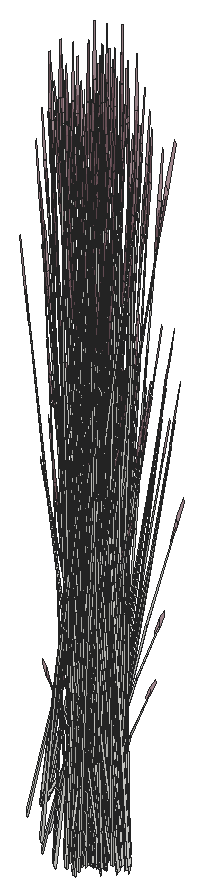
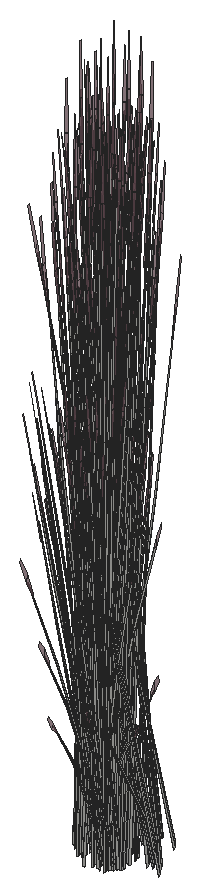
# SketchUp Ruby script. Lengths in inches.
U = 1.inch
M = Sketchup.active_model
def pt(a) = Geom::Point3d.new(a.map { |v| v * U })
def face(e, loops, mat)
  f = e.add_face(loops[0].map { |a| pt(a) })
  loops[1..].each { |l| e.add_face(l.map { |a| pt(a) }).erase! }
  f.material = f.back_material = mat if mat
  f
end
# faces: each face lists its corners as indices into pts; further lists are holes
def faces(e, pts, list, mat = nil) = list.each { |f| face(e, (f[0].is_a?(Array) ? f : [f]).map { |l| l.map { |i| pts[i] } }, mat) }
# xy, xz, yz: faces in a plane at the given z, y or x. An outline is a flat list of corners, or four numbers for a rectangle; further outlines are holes
def ring(l) = l.size == 4 ? [[l[0], l[1]], [l[2], l[1]], [l[2], l[3]], [l[0], l[3]]] : l.each_slice(2).to_a
def flat(e, list, mat, &to3) = list.each { |f| face(e, (f[0].is_a?(Array) ? f : [f]).map { |l| ring(l).map { |u, v| to3.(u, v) } }, mat) }
def xy(e, z, list, mat = nil) = flat(e, list, mat) { |x, y| [x, y, z] }
def xz(e, y, list, mat = nil) = flat(e, list, mat) { |x, z| [x, y, z] }
def yz(e, x, list, mat = nil) = flat(e, list, mat) { |y, z| [x, y, z] }
def lines(e, pts, list) = list.each { |a, b| e.add_line(pt(pts[a]), pt(pts[b])) }
# prism: a flat outline (further loops are holes) pulled along v
def prism(e, loops, v, mat = nil)
  f = face(e, loops, mat); d = Geom::Vector3d.new(v.map { |x| x * U })
  f.pushpull(f.normal.samedirection?(d) ? d.length : -d.length)
end
def box(e, o, s, mat = nil) = prism(e, [[o, [o[0] + s[0], o[1], o[2]], [o[0] + s[0], o[1] + s[1], o[2]], [o[0], o[1] + s[1], o[2]]]], [0, 0, s[2]], mat)
def at(x, y, z, deg = 0) = Geom::Transformation.translation(pt([x, y, z])) * Geom::Transformation.rotation(ORIGIN, Z_AXIS, deg.degrees)
def axes(o, x, y, z) = Geom::Transformation.new([*x, 0, *y, 0, *z, 0, *pt(o).to_a, 1])
def part(name) = M.definitions.add(name)
# library, detail: a bought-in or finely detailed component or shape, given as its bounding box
def library(name, o, s) = part(name).tap { |d| box(d.entities, o, s) }
def detail(e, o, s) = box(e.add_group.entities, o, s)
def put(e, d, t, mat = nil) = e.add_instance(d, t).tap { |i| i.material = mat if mat }
def group(e, t, mat = nil) = e.add_group.tap { |g| g.transformation = t; g.material = mat if mat }.entities
root = M.entities
M.materials.add("LightPink_Translucent").color = [144, 107, 117]
M.materials["LightPink_Translucent"].alpha = 0.75
c1 = part("blade")
p = [[2.15,0.21,22],[0,0.17,0],[0.09,0.45,0],[2.18,0.31,22],[2.29,0.31,22],[0.38,0.45,0],
  [2.48,0.24,33],[2.49,0.24,33],[2.48,0.22,33]]
faces(c1.entities,p,[[0,1,2,3],[4,5,2,3],[6,3,4,7],[8,0,3,6]])
c2 = part("seeds")
p = [[0.3,-0.1,1.38],[-0.01,-0.03,1.59],[-0.01,-0.03,0.03],[0.14,-0.07,-0.07],[0.29,-0.03,3],[0.15,0.01,3.11]]
faces(c2.entities,p,[[0,1,2,3],[1,0,4,5]],"LightPink_Translucent")
c3 = part("blade with seeds")
put(c3.entities,c1,at(0,0,0))
put(c3.entities,c2,axes([2.4,0.25,30.99],[1.5799,-0.05474,1.17369],[-0.12525,1.92788,0.29478],[-0.07173,-0.02425,1.56792]))
put(root,c3,axes([340.1,651.66,621.58],[0.44609,0.09826,0.45755],[-0.09078,0.55493,0.17955],[-0.06519,-0.05359,1.58856]))
put(root,c3,axes([337.55,651.78,624.45],[0.12963,0.31798,0.0643],[-0.23638,0.15564,0.50621],[0.1042,-0.03071,0.77189]))
put(root,c3,axes([337.24,652.63,624.25],[0.20082,0.29199,-0.35414],[-0.2293,0.2764,0.4572],[0.1165,0.04206,0.87481]))
put(root,c3,axes([341.33,650.97,624.76],[0.29332,0.1301,0.35414],[-0.08555,0.37955,-0.4572],[-0.11809,0.0348,0.87481]))
put(root,c3,axes([341.72,652.06,621.78],[-0.34464,-0.37536,-0.25192],[0.29,-0.42149,0.5513],[-0.0928,0.04391,1.68216]))
put(root,c3,axes([337.01,652.66,624.76],[0.0189,-0.47427,-0.1216],[0.35781,0.01296,-0.67495],[0.13781,0.03295,1.02557]))
put(root,c3,axes([337.53,651.66,624.46],[-0.09971,0.42522,0.48003],[-0.32782,-0.1454,0.3958],[0.12892,-0.02555,0.9933]))
put(root,c3,axes([341.38,652.15,624.39],[0.09067,0.42583,-0.51099],[-0.34336,0.07449,-0.3958],[-0.0984,0.11438,0.97773]))
put(root,c3,axes([339.98,651.55,621.94],[-0.17124,0.42022,0.44739],[-0.35581,-0.20224,-0.21531],[0,-0.09687,1.43643]))
put(root,c3,axes([342.24,651.85,621.77],[-0.36714,-0.07646,-0.62353],[0.07747,-0.47163,-0.16365],[-0.10956,-0.05715,1.37633]))
put(root,c3,axes([341.54,651.98,621.53],[-0.38326,0.02879,-0.44739],[-0.03466,-0.47788,0.21531],[-0.06861,0.04843,1.43643]))
put(root,c3,axes([339.86,652.54,621.7],[0.37926,-0.12378,0.17642],[0.09365,0.46065,0.35086],[-0.03382,-0.06712,1.60407]))
put(root,c3,axes([343.14,651.43,623.6],[0.12246,-0.09864,1.71376],[0.1031,0.45582,0.13857],[-0.19225,0.10302,0.73262]))
put(root,c3,axes([340.35,652.61,621.42],[-0.35581,-0.20937,0],[0.17124,-0.43505,0],[0,0,1.62707]))
put(root,c3,axes([340.8125,652.78,621.8],[0.33032,0.23318,0.49651],[-0.19744,0.41812,0],[-0.07523,-0.05311,1.57504]))
put(root,c3,axes([341.17,653.14,621.6],[0.22066,0.46731,0],[-0.36918,0.26061,-0.51607],[-0.08408,0.05936,1.63711]))
put(root,c3,axes([337.32,652.38,624.4375],[0.07571,-0.00789,1.74944],[0.20767,-0.36231,-0.27667],[0.13467,0.04783,0.14031]))
put(root,c3,axes([342.76,652.2,622.32],[0.12266,0.03828,1.43002],[0.07906,0.39104,-0.30754],[-0.16661,0.0732,0.61141]))
put(root,c3,axes([341.76,652.74,621.72],[-0.33032,-0.23318,-0.49651],[0.19744,-0.41812,0],[-0.07523,-0.05311,1.57504]))
put(root,c3,axes([341.22,651.85,624.74],[0.32648,0.25715,-0.1216],[-0.18809,0.3724,-0.67495],[-0.09224,0.12945,1.02557]))
put(root,c3,axes([338.22,651.7,622.49],[-0.21807,0.07699,1.1486],[0.10265,-0.31819,0.84392],[0.11568,0.02177,0.25299]))
put(root,c3,axes([341.28,652.05,621.93],[-0.06809,0.4162,0.1448],[-0.33266,-0.07225,-0.41347],[-0.06054,-0.04274,1.26744]))
put(root,c3,axes([341.96,653.02,622.08],[-0.22066,0.46731,0],[-0.36918,-0.26061,-0.51607],[-0.08408,-0.05936,1.63711]))
put(root,c3,axes([340.99,652.57,621.7],[0.10196,-0.46348,0.17642],[0.3731,0.13116,0.35086],[-0.06445,0.00226,1.60407]))
put(root,c3,axes([340.8125,651.95,621.84],[0.26075,0.2802,0.1448],[-0.2175,0.31612,-0.41347],[-0.06054,0.04274,1.26744]))
put(root,c3,axes([343.85,650.95,623.07],[0.10032,-0.06746,1.77064],[0.0346,0.47103,0.13857],[-0.2173,0.0625,0.63284]))
put(root,c3,axes([341.95,653.21,621.33],[-0.33032,0.23318,-0.49651],[-0.19744,-0.41812,0],[-0.07523,0.05311,1.57504]))
put(root,c3,axes([341.97,653.09,621.51],[-0.21791,-0.46895,-0.05142],[0.36918,-0.26061,0.51607],[-0.09097,0.04465,1.6363]))
put(root,c3,axes([340.72,651.61,621.52],[-0.32829,-0.4014,-0.06131],[0.32849,-0.40164,0],[-0.01146,-0.01402,1.75571]))
put(root,c3,axes([340.81,651.75,621.94],[0.38326,-0.02879,0.44739],[0.03466,0.47788,-0.21531],[-0.06861,0.04843,1.43643]))
put(root,c3,axes([337.59,651.62,624.25],[0.29332,0.1301,-0.35414],[-0.08555,0.37955,0.4572],[0.11809,-0.0348,0.87481]))
put(root,c3,axes([340.68,652.96,625.35],[0.31145,0.12449,-0.06488],[-0.0958,0.38314,-0.29416],[-0.05094,0.05817,0.97024]))
put(root,c3,axes([340.9,652.85,621.55],[0.44186,0.15158,0.30756],[-0.11054,0.54181,-0.36492],[-0.07313,0.06781,1.64885]))
put(root,c3,axes([341.87,653.03,621.35],[-0.32928,-0.11539,-0.30978],[0.08291,-0.40636,0.30978],[-0.06638,0.04686,1.38974]))
put(root,c3,axes([340.46,652.64,624.37],[0.23881,-0.24554,0.35414],[0.22606,0.28036,-0.4572],[-0.0344,0.14245,0.87481]))
put(root,c3,axes([337.03,652.4375,624.71],[0.35281,0.01123,-0.71045],[-0.0237,0.47284,0.08574],[0.14947,0.0499,1.00501]))
put(root,c3,axes([341.38,651.88,624.76],[0.30722,-0.06665,0.35414],[0.08112,0.381,-0.4572],[-0.08804,0.10234,0.87481]))
put(root,c3,axes([341.09,652.82,621.7],[0.33032,-0.23318,0.49651],[0.19744,0.41812,0],[-0.07523,0.05311,1.57504]))
put(root,c3,axes([342.06,651.29,622.16],[-0.00964,-0.43909,1.41272],[0.43635,0.11382,0.59816],[-0.1032,0.24027,1.3335]))
put(root,c3,axes([337.74,651.54,621.71],[-0.22732,0.05597,1.41583],[-0.03618,-0.44548,0.08104],[0.15921,-0.06743,0.80566]))
put(root,c3,axes([342.77,651.27,624.44],[-0.05763,0.06055,1.74944],[0.0049,0.44239,-0.27667],[-0.13211,0.05753,0.14031]))
put(root,c3,axes([340.43,652.43,621.43],[-0.11516,-0.40207,0],[0.32884,-0.1408,0],[0,0,1.54371]))
put(root,c3,axes([337.99,651.25,621.22],[-0.01845,-0.0708,1.76342],[0.12793,-0.41416,-0.26939],[0.12905,-0.00596,0.30037]))
put(root,c3,axes([338.12,653.04,624.43],[-0.03191,-0.04083,1.77383],[0.06981,-0.43764,-0.16761],[0.12571,-0.02796,0.31391]))
put(root,c3,axes([336.8,651.15,623.6],[-0.14639,0.01056,1.71376],[0.09712,-0.45778,0.13857],[0.20862,0.02831,0.73262]))
put(root,c3,axes([342.95,651.01,624.25],[-0.29332,-0.1301,-0.35414],[0.08555,-0.37955,0.4572],[-0.11809,0.0348,0.87481]))
put(root,c3,axes([341.8125,651.85,621.98],[0.04113,0.53214,-0.29095],[-0.42835,0.03218,-0.50002],[-0.07543,0.07088,1.59708]))
put(root,c3,axes([342.65,651.92,622.375],[-0.35635,0.30962,-0.29095],[-0.23697,-0.43749,-0.50002],[-0.08792,-0.04443,1.59708]))
put(root,c3,axes([341.67,652.89,624.44],[-0.25132,-0.3182,0.48003],[0.2669,-0.27442,0.3958],[-0.04636,0.14929,0.9933]))
put(root,c3,axes([337.33,651.58,624.71],[0.31014,-0.20596,-0.71045],[0.17284,0.42397,0.08574],[0.14985,-0.04816,1.00501]))
put(root,c3,axes([342.13,651.71,624.43],[0.04504,0.01251,1.77383],[0.13934,0.41205,-0.16761],[-0.0922,0.10815,0.31391]))
put(root,c3,axes([343.15,651.21,624.41],[-0.09562,0.42421,-0.51099],[-0.32782,-0.1454,-0.3958],[-0.13199,0.0389,0.97773]))
put(root,c3,axes([340.89,651.64,621.43],[-0.17124,0.42022,-0.44739],[-0.35581,-0.20224,0.21531],[0,0.09687,1.43643]))
put(root,c3,axes([341.85,652.57,621.74],[-0.08291,-0.40636,-0.30978],[0.32928,-0.11539,0.30978],[-0.06638,-0.04686,1.38974]))
put(root,c3,axes([341.58,652.86,624.4375],[-0.29004,-0.02173,0.0643],[0.00795,-0.32812,0.50621],[-0.03035,0.12569,0.77189]))
put(root,c3,axes([341.17,651.66,621.68],[0.44609,0.09826,0.45755],[-0.09078,0.55493,0.17955],[-0.06519,-0.05359,1.58856]))
put(root,c3,axes([342.99,651.18,621.22],[0.00895,0.0735,1.76342],[-0.18044,0.38382,-0.26939],[-0.12817,-0.01935,0.30037]))
put(root,c3,axes([341.57,651.38,621.7],[-0.2773,-0.3397,0.17642],[0.27945,-0.32949,0.35086],[-0.03063,0.06937,1.60407]))
put(root,c3,axes([340.61,651.1875,621.43],[0,-0.53961,0],[0.44133,0,0],[0,0,1.79456]))
put(root,c3,axes([341.06,651.55,622.04],[-0.17124,0.42022,0.44739],[-0.35581,-0.20224,-0.21531],[0,-0.09687,1.43643]))
put(root,c3,axes([340.83,651.4,621.52],[0,0.53934,-0.05637],[-0.44133,0,0],[0,0.01695,1.79368]))
put(root,c3,axes([342.89,652.25,621.77],[-0.23773,0.35053,-0.62353],[-0.29532,-0.31785,-0.16365],[-0.09526,0.08744,1.37633]))
put(root,c3,axes([340.05,653.05,624.28],[0.1064,-0.35863,0.35414],[0.31043,0.1046,-0.4572],[0.02846,0.14439,0.87481]))
put(root,c3,axes([342.51,653.02,622.49],[0.14709,-0.21136,1.1486],[0.05804,0.3346,0.84392],[-0.1063,0.05991,0.25299]))
put(root,c3,axes([337.81,652.21,622.31],[-0.085,-0.1147,1.43002],[0.1106,-0.37943,-0.30754],[0.17198,0.0514,0.61141]))
put(root,c3,axes([339.89,650.15,621.7],[-0.10196,0.46348,0.17642],[-0.3731,-0.13116,0.35086],[0.06445,-0.00226,1.60407]))
put(root,c3,axes([340.62,652.45,621.52],[0.15345,0.53576,-0.06012],[-0.43845,0.18773,0],[0.00536,0.01871,1.72173]))
put(root,c3,axes([340.94,652.54,621.79],[0.37926,-0.12378,0.17642],[0.09365,0.46065,0.35086],[-0.03382,-0.06712,1.60407]))
put(root,c3,axes([343.02,650.97,624.46],[0.09971,-0.42522,0.48003],[0.32782,0.1454,0.3958],[-0.12892,0.02555,0.9933]))
put(root,c3,axes([343.14,650.84,624.76],[0.17758,0.42229,-0.1216],[-0.31518,0.20752,-0.67495],[-0.13282,0.05572,1.02557]))
put(root,c3,axes([343.05,652.06,622.17],[-0.34464,-0.37536,-0.25192],[0.29,-0.42149,0.5513],[-0.0928,0.04391,1.68216]))
put(root,c3,axes([341.42,652.61,621.51],[-0.35581,-0.20937,0],[0.17124,-0.43505,0],[0,0,1.62707]))
put(root,c3,axes([342.25,653.14,621.69],[0.22066,0.46731,0],[-0.36918,0.26061,-0.51607],[-0.08408,0.05936,1.63711]))
put(root,c3,axes([343,650.85,624.46],[-0.12963,-0.31798,0.0643],[0.23638,-0.15564,0.50621],[-0.1042,0.03071,0.77189]))
put(root,c3,axes([343.59,651.73,623.6],[0.08815,-0.14329,1.71376],[0.22258,0.38678,0.13857],[-0.15267,0.17614,0.73262]))
put(root,c3,axes([341.89,651.74,621.42],[-0.44111,-0.00373,-0.04976],[0,-0.52122,0.49943],[-0.01386,0.11865,1.58352]))
put(root,c3,axes([343.0625,652.11,624.25],[-0.30722,0.06665,-0.35414],[-0.08112,-0.381,0.4572],[-0.08804,0.10234,0.87481]))
put(root,c3,axes([341.02,650.18,621.7],[-0.37926,0.12378,0.17642],[-0.09365,-0.46065,0.35086],[0.03382,0.06712,1.60407]))
put(root,c3,axes([342.88,651.98,621.92],[-0.38326,0.02879,-0.44739],[-0.03466,-0.47788,0.21531],[-0.06861,0.04843,1.43643]))
put(root,c3,axes([342.89,653.24,621.22],[0.04734,0.04659,1.76342],[0.08027,0.4317,-0.26939],[-0.10492,0.09206,0.30037]))
put(root,c3,axes([342.0625,652.57,621.79],[0.10196,-0.46348,0.17642],[0.3731,0.13116,0.35086],[-0.06445,0.00226,1.60407]))
put(root,c3,axes([341.89,651.95,621.93],[0.26075,0.2802,0.1448],[-0.2175,0.31612,-0.41347],[-0.06054,0.04274,1.26744]))
put(root,c3,axes([340.47,654.32,624.87],[0.2439,-0.26754,-0.06488],[0.22348,0.29302,-0.29416],[0.01573,0.08303,0.97024]))
put(root,c3,axes([340.4,650.85,621.58],[-0.29264,0.42323,0.45755],[-0.34767,-0.3736,0.17955],[0.07055,-0.04224,1.58856]))
put(root,c3,axes([341.8,651.61,621.61],[-0.32829,-0.4014,-0.06131],[0.32849,-0.40164,0],[-0.01146,-0.01402,1.75571]))
put(root,c3,axes([341.89,651.75,622.04],[0.38326,-0.02879,0.44739],[0.03466,0.47788,-0.21531],[-0.06861,0.04843,1.43643]))
put(root,c3,axes([340.9,651.52,621.4375],[0.24637,0.30123,0],[-0.24637,0.30123,0],[0,0,1.69266]))
put(root,c3,axes([343.1,652.03,624.46],[-0.08753,-0.42921,0.48003],[0.34336,-0.07449,0.3958],[-0.1012,0.10094,0.9933]))
put(root,c3,axes([340.9,651.16,621.94],[0.17124,-0.42022,0.44739],[0.35581,0.20224,-0.21531],[0,0.09687,1.43643]))
put(root,c3,axes([342.15,652.78,622.1875],[0.33032,0.23318,0.49651],[-0.19744,0.41812,0],[-0.07523,-0.05311,1.57504]))
put(root,c3,axes([340.75,652.62,621.43],[0.35581,0.20937,0],[-0.17124,0.43505,0],[0,0,1.74954]))
put(root,c3,axes([341.98,652.85,621.65],[0.44186,0.15158,0.30756],[-0.11054,0.54181,-0.36492],[-0.07313,0.06781,1.64885]))
put(root,c3,axes([343.03,651.94,624.46],[-0.2423,-0.19613,0.0643],[0.14107,-0.2793,0.50621],[-0.07768,0.0903,0.77189]))
put(root,c3,axes([342.17,652.82,621.8],[0.33032,-0.23318,0.49651],[0.19744,0.41812,0],[-0.07523,0.05311,1.57504]))
put(root,c3,axes([340.78,651.0625,621.61],[-0.44609,-0.09826,0.49198],[0.09078,-0.55493,0.19306],[0.06519,0.05359,1.70813]))
put(root,c3,axes([342.62,652.05,622.32],[-0.06809,0.4162,0.1448],[-0.33266,-0.07225,-0.41347],[-0.06054,-0.04274,1.26744]))
put(root,c3,axes([341.8,651.82,621.25],[-0.24637,0.29097,-0.30978],[-0.24637,-0.29097,0.30978],[0,0.09372,1.38974]))
put(root,c3,axes([343.28,653.21,621.72],[-0.33032,0.23318,-0.49651],[-0.19744,-0.41812,0],[-0.07523,0.05311,1.57504]))
put(root,c3,axes([341.5,652.43,621.52],[-0.11516,-0.40207,0],[0.32884,-0.1408,0],[0,0,1.54371]))
put(root,c3,axes([343.3,653.09,621.9],[-0.21791,-0.46895,-0.05142],[0.36918,-0.26061,0.51607],[-0.09097,0.04465,1.6363]))
put(root,c3,axes([343.53,652.09,623.6],[0.06572,-0.16029,1.71376],[0.27569,0.33172,0.13857],[-0.12437,0.20675,0.73262]))
put(root,c3,axes([341.09,651.77,621.32],[0.12941,0.42699,-0.69212],[-0.37279,0.15378,-0.18165],[0.0143,0.14459,1.52773]))
put(root,c3,axes([340.91,651.31,621.43],[0.39487,0,0],[0,0.48281,0],[0,0,1.78407]))
put(root,c3,axes([343.26,650.97,624.78],[0.29332,0.1301,0.35414],[-0.08555,0.37955,-0.4572],[-0.11809,0.0348,0.87481]))
put(root,c3,axes([340.53,650.78,621.94],[-0.21202,-0.39143,0.44739],[0.32115,-0.27564,-0.21531],[0.06861,0.04843,1.43643]))
put(root,c3,axes([343.2,653.03,621.74],[-0.32928,-0.11539,-0.30978],[0.08291,-0.40636,0.30978],[-0.06638,0.04686,1.38974]))
put(root,c3,axes([341.05,651.26,621.84],[0.32884,-0.136,0.1448],[0.11516,0.38837,-0.41347],[0,0.08547,1.26744]))
put(root,c3,axes([341.79,652.64,624.76],[0.23881,-0.24554,0.35414],[0.22606,0.28036,-0.4572],[-0.0344,0.14245,0.87481]))
put(root,c3,axes([343.3125,652.15,624.41],[0.09067,0.42583,-0.51099],[-0.34336,0.07449,-0.3958],[-0.0984,0.11438,0.97773]))
put(root,c3,axes([343.39,651.29,622.55],[-0.00964,-0.43909,1.41272],[0.43635,0.11382,0.59816],[-0.1032,0.24027,1.3335]))
put(root,c3,axes([341.97,651.64,621.53],[-0.17124,0.42022,-0.44739],[-0.35581,-0.20224,0.21531],[0,0.09687,1.43643]))
put(root,c3,axes([344.17,651.85,621.78],[-0.36714,-0.07646,-0.62353],[0.07747,-0.47163,-0.16365],[-0.10956,-0.05715,1.37633]))
put(root,c3,axes([340.93,651.29,621.89],[0.39748,0.22252,-0.29095],[-0.19139,0.46966,-0.50002],[0.01249,0.11531,1.59708]))
put(root,c3,axes([342.65,651.38,621.79],[-0.2773,-0.3397,0.17642],[0.27945,-0.32949,0.35086],[-0.03063,0.06937,1.60407]))
put(root,c3,axes([343.15,651.85,622.375],[0.04113,0.53214,-0.29095],[-0.42835,0.03218,-0.50002],[-0.07543,0.07088,1.59708]))
put(root,c3,axes([341.6875,651.1875,621.52],[0,-0.53961,0],[0.44133,0,0],[0,0,1.79456]))
put(root,c3,axes([341.91,651.4,621.61],[0,0.53934,-0.05637],[-0.44133,0,0],[0,0.01695,1.79368]))
put(root,c3,axes([341.13,653.05,624.37],[0.1064,-0.35863,0.35414],[0.31043,0.1046,-0.4572],[0.02846,0.14439,0.87481]))
put(root,c3,axes([341.8,651.4,621.7],[0,-0.46636,0.49651],[0.39487,0,0],[0,0.10622,1.57504]))
put(root,c3,axes([341.97,651.83,621.24],[0,0.46636,-0.49651],[-0.39487,0,0],[0,0.10622,1.57504]))
put(root,c3,axes([340.91,653.24,623.96],[-0.35104,0.10702,0.48003],[-0.06092,-0.41983,0.3958],[0.08256,0.12373,0.9933]))
put(root,c3,axes([343.6875,652.74,621.74],[-0.33032,-0.23318,-0.49651],[0.19744,-0.41812,0],[-0.07523,-0.05311,1.57504]))
put(root,c3,axes([340.84,653.33,623.95],[-0.16041,0.29625,0.0643],[-0.22843,-0.17248,0.50621],[0.07385,0.09498,0.77189]))
put(root,c3,axes([340.97,650.15,621.79],[-0.10196,0.46348,0.17642],[-0.3731,-0.13116,0.35086],[0.06445,-0.00226,1.60407]))
put(root,c3,axes([343.15,651.85,624.76],[0.32648,0.25715,-0.1216],[-0.18809,0.3724,-0.67495],[-0.09224,0.12945,1.02557]))
put(root,c3,axes([341.7,652.45,621.61],[0.15345,0.53576,-0.06012],[-0.43845,0.18773,0],[0.00536,0.01871,1.72173]))
put(root,c3,axes([340.67,650.67,621.84],[0.06809,-0.4162,0.1448],[0.33266,0.07225,-0.41347],[0.06054,0.04274,1.26744]))
put(root,c3,axes([342.51,651.66,622.07],[0.44609,0.09826,0.45755],[-0.09078,0.55493,0.17955],[-0.06519,-0.05359,1.58856]))
put(root,c3,axes([343.89,653.02,622.1],[-0.22066,0.46731,0],[-0.36918,-0.26061,-0.51607],[-0.08408,-0.05936,1.63711]))
put(root,c3,axes([341.15,649.94,621.7],[-0.33032,-0.23318,0.49651],[0.19744,-0.41812,0],[0.07523,0.05311,1.57504]))
put(root,c3,axes([342.39,651.55,622.43],[-0.17124,0.42022,0.44739],[-0.35581,-0.20224,-0.21531],[0,-0.09687,1.43643]))
put(root,c3,axes([342.97,651.74,621.52],[-0.44111,-0.00373,-0.04976],[0,-0.52122,0.49943],[-0.01386,0.11865,1.58352]))
put(root,c3,axes([342.61,652.96,625.37],[0.31145,0.12449,-0.06488],[-0.0958,0.38314,-0.29416],[-0.05094,0.05817,0.97024]))
put(root,c3,axes([342.1,650.18,621.79],[-0.37926,0.12378,0.17642],[-0.09365,-0.46065,0.35086],[0.03382,0.06712,1.60407]))
put(root,c3,axes([340.86,652.375,621.41],[0.37054,-0.15823,-0.19198],[0.1302,0.45581,0.00008],[0.0409,-0.01749,1.73897]))
put(root,c3,axes([343.3125,651.88,624.78],[0.30722,-0.06665,0.35414],[0.08112,0.381,-0.4572],[-0.08804,0.10234,0.87481]))
put(root,c3,axes([342.27,652.54,622.18],[0.37926,-0.12378,0.17642],[0.09365,0.46065,0.35086],[-0.03382,-0.06712,1.60407]))
put(root,c3,axes([341.55,654.32,624.96],[0.2439,-0.26754,-0.06488],[0.22348,0.29302,-0.29416],[0.01573,0.08303,0.97024]))
put(root,c3,axes([341.48,650.85,621.68],[-0.29264,0.42323,0.45755],[-0.34767,-0.3736,0.17955],[0.07055,-0.04224,1.58856]))
put(root,c3,axes([342.76,652.61,621.9],[-0.35581,-0.20937,0],[0.17124,-0.43505,0],[0,0,1.62707]))
put(root,c3,axes([341.98,651.52,621.53],[0.24637,0.30123,0],[-0.24637,0.30123,0],[0,0,1.69266]))
put(root,c3,axes([340.79,652.99,624.28],[-0.05451,-0.37564,0.35414],[0.31161,-0.09919,-0.4572],[0.0837,0.10765,0.87481]))
put(root,c3,axes([341.98,651.16,622.04],[0.17124,-0.42022,0.44739],[0.35581,0.20224,-0.21531],[0,0.09687,1.43643]))
put(root,c3,axes([343.58,653.14,622.08],[0.22066,0.46731,0],[-0.36918,0.26061,-0.51607],[-0.08408,0.05936,1.63711]))
put(root,c3,axes([341.83,652.62,621.52],[0.35581,0.20937,0],[-0.17124,0.43505,0],[0,0,1.74954]))
put(root,c3,axes([340.86,651.02,621.43],[0.21202,0.39143,-0.44739],[-0.32115,0.27564,0.21531],[0.06861,0.04843,1.43643]))
put(root,c3,axes([341,650.82,623.7],[-0.30498,-0.24231,1.38283],[0.32203,-0.37727,0.59665],[0.0984,0.22736,1.33663]))
put(root,c3,axes([341.86,651.0625,621.7],[-0.44609,-0.09826,0.49198],[0.09078,-0.55493,0.19306],[0.06519,0.05359,1.70813]))
put(root,c3,axes([344.59,651.92,622.39],[-0.35635,0.30962,-0.29095],[-0.23697,-0.43749,-0.50002],[-0.08792,-0.04443,1.59708]))
put(root,c3,axes([343.6,652.89,624.46],[-0.25132,-0.3182,0.48003],[0.2669,-0.27442,0.3958],[-0.04636,0.14929,0.9933]))
put(root,c3,axes([343.4,652.57,622.18],[0.10196,-0.46348,0.17642],[0.3731,0.13116,0.35086],[-0.06445,0.00226,1.60407]))
put(root,c3,axes([340.49,653.51,623.93],[0.00104,-0.05646,1.77383],[0.30246,-0.2491,-0.16761],[0.10506,0.08891,0.31391]))
put(root,c3,axes([343.23,651.95,622.32],[0.26075,0.2802,0.1448],[-0.2175,0.31612,-0.41347],[-0.06054,0.04274,1.26744]))
put(root,c3,axes([342.875,651.82,621.35],[-0.24637,0.29097,-0.30978],[-0.24637,-0.29097,0.30978],[0,0.09372,1.38974]))
put(root,c3,axes([341.46,652.8,621.99],[-0.19872,-0.13409,1.1486],[0.2566,-0.13625,0.84392],[0.06921,0.11541,0.25299]))
put(root,c3,axes([340.76,652.65,621.81],[0.00623,-0.15459,1.43002],[0.29764,-0.17268,-0.30754],[0.09188,0.18503,0.61141]))
put(root,c3,axes([343.13,651.61,622],[-0.32829,-0.4014,-0.06131],[0.32849,-0.40164,0],[-0.01146,-0.01402,1.75571]))
put(root,c3,axes([343.78,652.57,621.75],[-0.08291,-0.40636,-0.30978],[0.32928,-0.11539,0.30978],[-0.06638,-0.04686,1.38974]))
put(root,c3,axes([343.22,651.75,622.43],[0.38326,-0.02879,0.44739],[0.03466,0.47788,-0.21531],[-0.06861,0.04843,1.43643]))
put(root,c3,axes([342.17,651.77,621.41],[0.12941,0.42699,-0.69212],[-0.37279,0.15378,-0.18165],[0.0143,0.14459,1.52773]))
put(root,c3,axes([343.51,652.86,624.46],[-0.29004,-0.02173,0.0643],[0.00795,-0.32812,0.50621],[-0.03035,0.12569,0.77189]))
put(root,c3,axes([341.99,651.31,621.52],[0.39487,0,0],[0,0.48281,0],[0,0,1.78407]))
put(root,c3,axes([343.3125,652.85,622.04],[0.44186,0.15158,0.30756],[-0.11054,0.54181,-0.36492],[-0.07313,0.06781,1.64885]))
put(root,c3,axes([341.61,650.78,622.04],[-0.21202,-0.39143,0.44739],[0.32115,-0.27564,-0.21531],[0.06861,0.04843,1.43643]))
put(root,c3,axes([342.125,651.26,621.93],[0.32884,-0.136,0.1448],[0.11516,0.38837,-0.41347],[0,0.08547,1.26744]))
put(root,c3,axes([343.5,652.82,622.1875],[0.33032,-0.23318,0.49651],[0.19744,0.41812,0],[-0.07523,0.05311,1.57504]))
put(root,c3,axes([344.82,652.25,621.78],[-0.23773,0.35053,-0.62353],[-0.29532,-0.31785,-0.16365],[-0.09526,0.08744,1.37633]))
put(root,c3,axes([341.44,650.15,621.25],[0.08291,0.40636,-0.30978],[-0.32928,0.11539,0.30978],[0.06638,0.04686,1.38974]))
put(root,c3,axes([342.06,651.48,621.6],[0.44133,0,0],[0,0.52122,-0.51607],[0,0.11871,1.63711]))
put(root,c3,axes([342.84,652.43,621.91],[-0.11516,-0.40207,0],[0.32884,-0.1408,0],[0,0,1.54371]))
put(root,c3,axes([342.01,651.29,621.98],[0.39748,0.22252,-0.29095],[-0.19139,0.46966,-0.50002],[0.01249,0.11531,1.59708]))
put(root,c3,axes([340.64,650.8,621.89],[0.35635,-0.30962,-0.29095],[0.23697,0.43749,-0.50002],[0.08792,0.04443,1.59708]))
put(root,c3,axes([341.5,653.41,621.89],[-0.22633,-0.01463,1.0506],[0.14947,-0.31064,0.58006],[0.08941,0.11036,0.8241]))
put(root,c3,axes([344.99,652.06,622.19],[-0.34464,-0.37536,-0.25192],[0.29,-0.42149,0.5513],[-0.0928,0.04391,1.68216]))
put(root,c3,axes([342.875,651.4,621.8],[0,-0.46636,0.49651],[0.39487,0,0],[0,0.10622,1.57504]))
put(root,c3,axes([343.04,651.83,621.33],[0,0.46636,-0.49651],[-0.39487,0,0],[0,0.10622,1.57504]))
put(root,c3,axes([341.99,653.24,624.05],[-0.35104,0.10702,0.48003],[-0.06092,-0.41983,0.3958],[0.08256,0.12373,0.9933]))
put(root,c3,axes([341.92,653.33,624.05],[-0.16041,0.29625,0.0643],[-0.22843,-0.17248,0.50621],[0.07385,0.09498,0.77189]))
put(root,c3,axes([343.3,651.64,621.92],[-0.17124,0.42022,-0.44739],[-0.35581,-0.20224,0.21531],[0,0.09687,1.43643]))
put(root,c3,axes([344.8125,651.98,621.9375],[-0.38326,0.02879,-0.44739],[-0.03466,-0.47788,0.21531],[-0.06861,0.04843,1.43643]))
put(root,c3,axes([341.75,650.67,621.93],[0.06809,-0.4162,0.1448],[0.33266,0.07225,-0.41347],[0.06054,0.04274,1.26744]))
put(root,c3,axes([340.77,653.18,624.26],[0.21031,-0.39918,-0.1216],[0.30457,0.22997,-0.67495],[0.10587,0.11278,1.02557]))
put(root,c3,axes([339.74,650.53,620.82],[-0.3474,0.18671,1.28929],[-0.11057,-0.53572,0.50096],[0.21332,0.00891,1.46642]))
put(root,c3,axes([343.98,651.38,622.18],[-0.2773,-0.3397,0.17642],[0.27945,-0.32949,0.35086],[-0.03063,0.06937,1.60407]))
put(root,c3,axes([343.02,651.1875,621.91],[0,-0.53961,0],[0.44133,0,0],[0,0,1.79456]))
put(root,c3,axes([342.22,649.94,621.8],[-0.33032,-0.23318,0.49651],[0.19744,-0.41812,0],[0.07523,0.05311,1.57504]))
put(root,c3,axes([344.08,652.78,622.2],[0.33032,0.23318,0.49651],[-0.19744,0.41812,0],[-0.07523,-0.05311,1.57504]))
put(root,c3,axes([343.24,651.4,622],[0,0.53934,-0.05637],[-0.44133,0,0],[0,0.01695,1.79368]))
put(root,c3,axes([342.46,653.05,624.76],[0.1064,-0.35863,0.35414],[0.31043,0.1046,-0.4572],[0.02846,0.14439,0.87481]))
put(root,c3,axes([341.02,652.98,623.9],[0.34827,-0.11086,-0.51099],[0.06092,0.41983,-0.3958],[0.09354,0.12031,0.97773]))
put(root,c3,axes([341.94,652.375,621.5],[0.37054,-0.15823,-0.19198],[0.1302,0.45581,0.00008],[0.0409,-0.01749,1.73897]))
put(root,c3,axes([342.31,650.15,622.18],[-0.10196,0.46348,0.17642],[-0.3731,-0.13116,0.35086],[0.06445,-0.00226,1.60407]))
put(root,c3,axes([343.03,652.45,622],[0.15345,0.53576,-0.06012],[-0.43845,0.18773,0],[0.00536,0.01871,1.72173]))
put(root,c3,axes([341.42,652.48,624.28],[-0.20082,-0.29199,0.35414],[0.2293,-0.2764,-0.4572],[0.1165,0.04206,0.87481]))
put(root,c3,axes([344.55,652.05,622.34],[-0.06809,0.4162,0.1448],[-0.33266,-0.07225,-0.41347],[-0.06054,-0.04274,1.26744]))
put(root,c3,axes([341.54,649.98,621.24],[0.33032,0.23318,-0.49651],[-0.19744,0.41812,0],[0.07523,0.05311,1.57504]))
